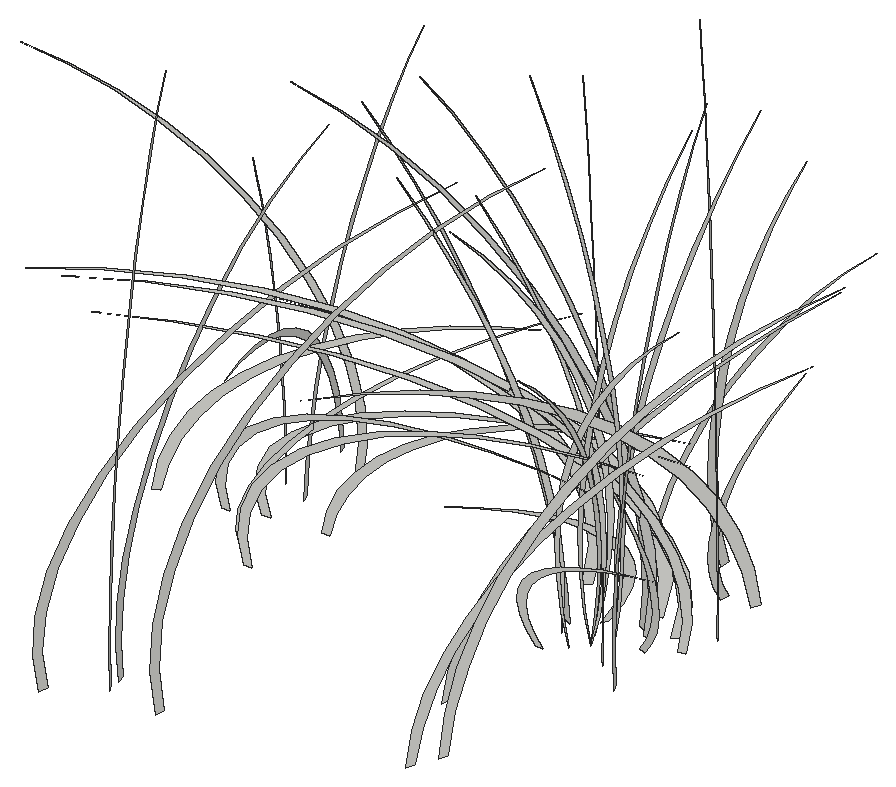
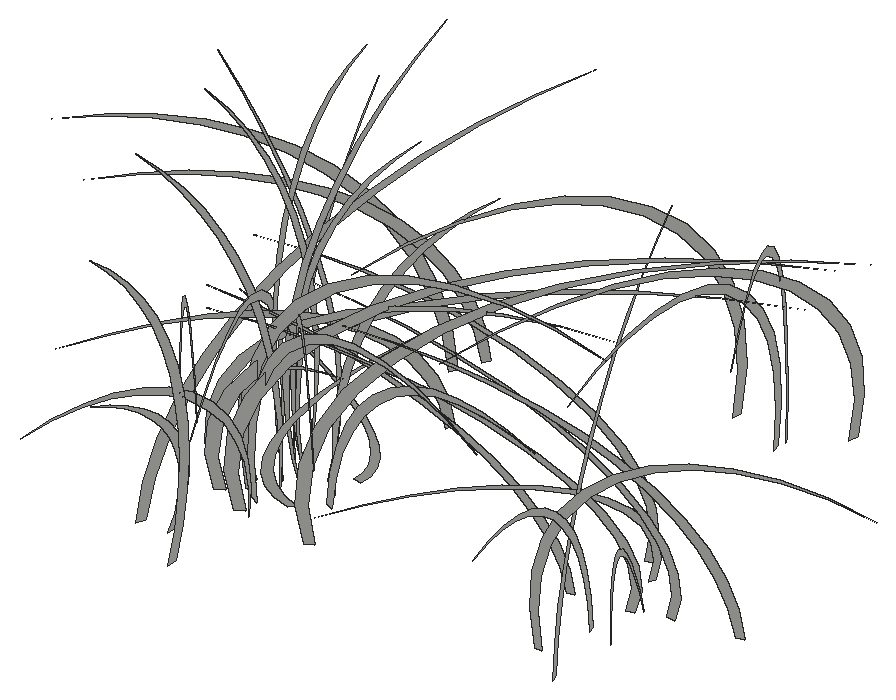
# SketchUp Ruby script. Lengths in inches.
U = 1.inch
M = Sketchup.active_model
def pt(a) = Geom::Point3d.new(a.map { |v| v * U })
def face(e, loops, mat)
  f = e.add_face(loops[0].map { |a| pt(a) })
  loops[1..].each { |l| e.add_face(l.map { |a| pt(a) }).erase! }
  f.material = f.back_material = mat if mat
  f
end
# faces: each face lists its corners as indices into pts; further lists are holes
def faces(e, pts, list, mat = nil) = list.each { |f| face(e, (f[0].is_a?(Array) ? f : [f]).map { |l| l.map { |i| pts[i] } }, mat) }
# xy, xz, yz: faces in a plane at the given z, y or x. An outline is a flat list of corners, or four numbers for a rectangle; further outlines are holes
def ring(l) = l.size == 4 ? [[l[0], l[1]], [l[2], l[1]], [l[2], l[3]], [l[0], l[3]]] : l.each_slice(2).to_a
def flat(e, list, mat, &to3) = list.each { |f| face(e, (f[0].is_a?(Array) ? f : [f]).map { |l| ring(l).map { |u, v| to3.(u, v) } }, mat) }
def xy(e, z, list, mat = nil) = flat(e, list, mat) { |x, y| [x, y, z] }
def xz(e, y, list, mat = nil) = flat(e, list, mat) { |x, z| [x, y, z] }
def yz(e, x, list, mat = nil) = flat(e, list, mat) { |y, z| [x, y, z] }
def lines(e, pts, list) = list.each { |a, b| e.add_line(pt(pts[a]), pt(pts[b])) }
# prism: a flat outline (further loops are holes) pulled along v
def prism(e, loops, v, mat = nil)
  f = face(e, loops, mat); d = Geom::Vector3d.new(v.map { |x| x * U })
  f.pushpull(f.normal.samedirection?(d) ? d.length : -d.length)
end
def box(e, o, s, mat = nil) = prism(e, [[o, [o[0] + s[0], o[1], o[2]], [o[0] + s[0], o[1] + s[1], o[2]], [o[0], o[1] + s[1], o[2]]]], [0, 0, s[2]], mat)
def at(x, y, z, deg = 0) = Geom::Transformation.translation(pt([x, y, z])) * Geom::Transformation.rotation(ORIGIN, Z_AXIS, deg.degrees)
def axes(o, x, y, z) = Geom::Transformation.new([*x, 0, *y, 0, *z, 0, *pt(o).to_a, 1])
def part(name) = M.definitions.add(name)
# library, detail: a bought-in or finely detailed component or shape, given as its bounding box
def library(name, o, s) = part(name).tap { |d| box(d.entities, o, s) }
def detail(e, o, s) = box(e.add_group.entities, o, s)
def put(e, d, t, mat = nil) = e.add_instance(d, t).tap { |i| i.material = mat if mat }
def group(e, t, mat = nil) = e.add_group.tap { |g| g.transformation = t; g.material = mat if mat }.entities
root = M.entities
g1 = group(root,at(67.39,563.36,0.02))
p = [[-0.5,0.78,0],[-0.22,0.34,0],[0,0,2.37],[-0.09,0.14,4.75],[-0.49,0.76,7.08],[-1.2,1.84,9.32],
  [-2.1875,3.37,11.39],[-3.4375,5.29,13.25],[-4.92,7.57,14.85],[-6.59,10.14,16.15],[-8.41,12.95,17.13],[-10.34,15.92,17.75],
  [-12.32,18.97,18.01],[-14.32,22.05,17.89],[-12.36,19.03,17.91],[-10.42,16.05,17.58],[-8.55,13.16,16.9],[-6.78,10.45,15.89],
  [-5.17,7.96,14.58],[-3.73,5.75,12.99],[-2.52,3.88,11.15],[-1.55,2.39,9.125],[-0.86,1.32,6.94],[-0.44,0.68,4.66],
  [-0.33,0.5,2.33]]
faces(g1,p,[[0,1,2,3,4,5,6,7,8,9,10,11,12,13,14,15,16,17,18,19,20,21,22,23,24]])
g2 = group(root,at(64.68,561.18,0.02))
p = [[0.08,0.99,0],[0.03,0.44,0],[0,0,2.01],[0.01,0.18,4.04],[0.08,0.97,6.02],[0.19,2.35,7.92],
  [0.34,4.3,9.68],[0.53,6.75,11.26],[0.76,9.66,12.62],[1.02,12.94,13.73],[1.3,16.52,14.5625],[1.6,20.31,15.09],
  [1.91,24.21,15.31],[2.21,28.13,15.2],[1.91,24.29,15.22],[1.61,20.48,14.94],[1.32,16.8,14.37],[1.05,13.33,13.51],
  [0.8,10.15,12.39],[0.58,7.34,11.04],[0.39,4.95,9.48],[0.24,3.05,7.75],[0.13,1.68,5.9],[0.07,0.87,3.96],
  [0.05,0.64,1.98]]
faces(g2,p,[[0,1,2,3,4,5,6,7,8,9,10,11,12,13,14,15,16,17,18,19,20,21,22,23,24]])
g3 = group(root,at(70.15,562.89,0.02))
p = [[0.07,0.92,0],[0.03,0.41,0],[0,0,2.37],[0.01,0.17,4.75],[0.07,0.9,7.08],[0.17,2.19,9.32],
  [0.32,4,11.39],[0.5,6.29,13.25],[0.71,9,14.85],[0.95,12.06,16.15],[1.21,15.39,17.13],[1.49,18.92,17.75],
  [1.78,22.55,18.01],[2.0625,26.21,17.89],[1.78,22.625,17.91],[1.5,19.08,17.58],[1.23,15.65,16.9],[0.98,12.42,15.89],
  [0.74,9.46,14.58],[0.54,6.84,12.99],[0.36,4.61,11.15],[0.22,2.84,9.125],[0.125,1.57,6.94],[0.0625,0.8125,4.66],
  [0.05,0.59,2.33]]
faces(g3,p,[[0,1,2,3,4,5,6,7,8,9,10,11,12,13,14,15,16,17,18,19,20,21,22,23,24]])
g4 = group(root,at(82.15,566.53,0.02))
p = [[7.01,17,14.81],[8.0625,19.56,15.2],[7.04,17.08,14.73],[6.05,14.68,14.07],[5.11,12.39,13.24],[4.22,10.24,12.25],
  [3.4,8.26,11.1],[2.66,6.45,9.81],[2,4.85,8.39],[1.43,3.47,6.86],[0.96,2.33,5.24],[0.59,1.4375,3.55],
  [0.33,0.81,1.79],[0.18,0.44,0],[0,0,0],[0.125,0.3,1.83],[0.37,0.89,3.63],[0.73,1.77,5.37],
  [1.2,2.92,7.03],[1.78,4.32,8.59],[2.46,5.97,10.02],[3.23,7.84,11.32],[4.08,9.91,12.46],[5,12.14,13.43],
  [5.98,14.51,14.21]]
faces(g4,p,[[0,1,2,3,4,5,6,7,8,9,10,11,12,13,14,15,16,17,18,19,20,21,22,23,24]])
g5 = group(root,at(67.11,564.21,0.02))
p = [[-0.27,0.88,0],[-0.12,0.39,0],[0,0,2.0625],[-0.05,0.16,4.13],[-0.26,0.87,6.16],[-0.64,2.1,8.1],
  [-1.17,3.84,9.91],[-1.84,6.03,11.52],[-2.64,8.63,12.92],[-3.54,11.5625,14.05],[-4.51,14.76,14.9],[-5.55,18.15,15.45],
  [-6.61,21.64,15.67],[-7.69,25.14,15.5625],[-6.63,21.7,15.58],[-5.59,18.3,15.29],[-4.59,15.01,14.71],[-3.64,11.91,13.83],
  [-2.77,9.07,12.68],[-2,6.56,11.3],[-1.35,4.43,9.7],[-0.83,2.73,7.9375],[-0.46,1.5,6.04],[-0.24,0.78,4.05],
  [-0.17,0.57,2.02]]
faces(g5,p,[[0,1,2,3,4,5,6,7,8,9,10,11,12,13,14,15,16,17,18,19,20,21,22,23,24]])
g6 = group(root,at(85.34,588.43,0.02))
p = [[-7.92,-19.21,16.73],[-9.11,-22.11,17.17],[-7.96,-19.3,16.64],[-6.84,-16.59,15.9],[-5.77,-14.01,14.96],[-4.77,-11.58,13.84],
  [-3.85,-9.33,12.54],[-3,-7.29,11.08],[-2.26,-5.48,9.48],[-1.62,-3.92,7.76],[-1.09,-2.63,5.92],[-0.67,-1.625,4.01],
  [-0.375,-0.91,2.02],[-0.21,-0.5,0],[0,0,0],[-0.14,-0.34,2.07],[-0.41,-1.01,4.1],[-0.82,-2,6.07],
  [-1.36,-3.3,7.94],[-2.01,-4.89,9.7],[-2.78,-6.75,11.33],[-3.65,-8.86,12.79],[-4.61,-11.19,14.08],[-5.65,-13.72,15.17],
  [-6.76,-16.4,16.0625]]
faces(g6,p,[[0,1,2,3,4,5,6,7,8,9,10,11,12,13,14,15,16,17,18,19,20,21,22,23,24]])
g7 = group(root,at(81.5,581.54,0.02))
p = [[0.19,-0.93,0],[0.09,-0.41,1.51],[0.02,-0.1,3.03],[0,0,4.56],[0.02,-0.1,6.09],[0.08,-0.41,7.61],
  [0.19,-0.92,9.12],[0.34,-1.63,10.61],[0.53,-2.55,12.07],[0.76,-3.65,13.5],[1.02,-4.95,14.89],[1.33,-6.43,16.24],
  [1.67,-8.09,17.53],[1.35,-6.53,16.21],[1.0625,-5.13,14.86],[0.81,-3.9,13.46],[0.59,-2.85,12.03],[0.41,-1.96,10.57],
  [0.26,-1.26,9.08],[0.15,-0.75,7.58],[0.08,-0.41,6.07],[0.05,-0.26,4.55],[0.0625,-0.3,3.03],[0.11,-0.52,1.51]]
faces(g7,p,[[0,1,2,3,4,5,6,7,8,9,10,11,12,13,14,15,16,17,18,19,20,21,22,23]])
g8 = group(root,at(78.48,585.41,0.02))
p = [[-0.76,-0.53,0],[-0.34,-0.24,0],[0,0,2.0625],[-0.14,-0.1,4.13],[-0.74,-0.52,6.16],[-1.8,-1.26,8.1],
  [-3.29,-2.3,9.91],[-5.18,-3.61,11.52],[-7.4,-5.16,12.92],[-9.92,-6.92,14.05],[-12.66,-8.83,14.9],[-15.56,-10.86,15.45],
  [-18.56,-12.94,15.67],[-21.56,-15.04,15.5625],[-18.61,-12.98,15.58],[-15.69,-10.95,15.29],[-12.875,-8.98,14.71],[-10.21,-7.125,13.83],
  [-7.78,-5.43,12.68],[-5.625,-3.92,11.3],[-3.8,-2.65,9.7],[-2.34,-1.63,7.9375],[-1.29,-0.9,6.04],[-0.67,-0.47,4.05],
  [-0.49,-0.34,2.02]]
faces(g8,p,[[0,1,2,3,4,5,6,7,8,9,10,11,12,13,14,15,16,17,18,19,20,21,22,23,24]])
g9 = group(root,at(78.48,585.41,0.02))
p = [[-0.76,-0.53,0],[-0.34,-0.24,0],[0,0,2.0625],[-0.14,-0.1,4.13],[-0.74,-0.52,6.16],[-1.8,-1.26,8.1],
  [-3.29,-2.3,9.91],[-5.18,-3.61,11.52],[-7.4,-5.16,12.92],[-9.92,-6.92,14.05],[-12.66,-8.83,14.9],[-15.56,-10.86,15.45],
  [-18.56,-12.94,15.67],[-21.56,-15.04,15.5625],[-18.61,-12.98,15.58],[-15.69,-10.95,15.29],[-12.875,-8.98,14.71],[-10.21,-7.125,13.83],
  [-7.78,-5.43,12.68],[-5.625,-3.92,11.3],[-3.8,-2.65,9.7],[-2.34,-1.63,7.9375],[-1.29,-0.9,6.04],[-0.67,-0.47,4.05],
  [-0.49,-0.34,2.02]]
faces(g9,p,[[0,1,2,3,4,5,6,7,8,9,10,11,12,13,14,15,16,17,18,19,20,21,22,23,24]])
g10 = group(root,at(82.8,568.11,0.02))
p = [[7.01,17,18.36],[8.0625,19.56,18.85],[7.04,17.08,18.26],[6.05,14.68,17.45],[5.11,12.39,16.42],[4.22,10.24,15.1875],
  [3.4,8.26,13.76],[2.66,6.45,12.16],[2,4.85,10.41],[1.43,3.47,8.51],[0.96,2.33,6.5],[0.59,1.4375,4.4],
  [0.33,0.81,2.22],[0.18,0.44,0],[0,0,0],[0.125,0.3,2.27],[0.37,0.89,4.5],[0.73,1.77,6.66],
  [1.2,2.92,8.72],[1.78,4.32,10.65],[2.46,5.97,12.43],[3.23,7.84,14.04],[4.08,9.91,15.45],[5,12.14,16.65],
  [5.98,14.51,17.625]]
faces(g10,p,[[0,1,2,3,4,5,6,7,8,9,10,11,12,13,14,15,16,17,18,19,20,21,22,23,24]])
g11 = group(root,at(64.3125,576.6,0.02))
p = [[0.76,0.1,0],[0.34,0.04,0],[0,0,1.44],[0.14,0.02,2.89],[0.74,0.09,4.3125],[1.8,0.23,5.67],
  [3.28,0.41,6.93],[5.15,0.65,8.0625],[7.37,0.93,9.04],[9.875,1.24,9.83],[12.61,1.59,10.43],[15.5,1.95,10.81],
  [18.47,2.33,10.96],[21.46,2.7,10.89],[18.53,2.33,10.9],[15.625,1.97,10.7],[12.82,1.61,10.29],[10.17,1.28,9.67],
  [7.75,0.98,8.875],[5.6,0.71,7.9],[3.78,0.48,6.79],[2.33,0.29,5.55],[1.28,0.16,4.22],[0.66,0.08,2.83],
  [0.49,0.0625,1.42]]
faces(g11,p,[[0,1,2,3,4,5,6,7,8,9,10,11,12,13,14,15,16,17,18,19,20,21,22,23,24]])
g12 = group(root,at(84.95,583.91,0.02))
p = [[-0.9,-0.41,0],[-0.4,-0.18,0],[0,0,1.75],[-0.16,-0.07,3.51],[-0.89,-0.4,5.24],[-2.15,-0.97,6.89],
  [-3.93,-1.77,8.42],[-6.17,-2.79,9.8],[-8.83,-3.99,10.98],[-11.83,-5.34,11.95],[-15.1,-6.82,12.67],[-18.57,-8.38,13.13],
  [-22.14,-9.99,13.32],[-25.72,-11.61,13.23],[-22.2,-10.03,13.25],[-18.72,-8.45,13],[-15.36,-6.93,12.5],[-12.1875,-5.5,11.75],
  [-9.28,-4.19,10.78],[-6.71,-3.03,9.6],[-4.53,-2.04,8.25],[-2.79,-1.26,6.75],[-1.54,-0.69,5.13],[-0.8,-0.36,3.44],
  [-0.58,-0.26,1.72]]
faces(g12,p,[[0,1,2,3,4,5,6,7,8,9,10,11,12,13,14,15,16,17,18,19,20,21,22,23,24]])
g13 = group(root,at(83.01,584.91,0.02))
p = [[-0.87,-0.48,0],[-0.39,-0.21,0],[0,0,2.01],[-0.16,-0.09,4.04],[-0.85,-0.47,6.02],[-2.07,-1.13,7.92],
  [-3.78,-2.07,9.68],[-5.94,-3.25,11.26],[-8.5,-4.65,12.62],[-11.39,-6.23,13.73],[-14.54,-7.96,14.5625],[-17.87,-9.78,15.09],
  [-21.3,-11.66,15.31],[-24.75,-13.55,15.2],[-21.37,-11.7,15.22],[-18.02,-9.86,14.94],[-14.78,-8.09,14.37],[-11.73,-6.42,13.51],
  [-8.93,-4.89,12.39],[-6.46,-3.53,11.04],[-4.36,-2.39,9.48],[-2.6875,-1.47,7.75],[-1.48,-0.8125,5.9],[-0.77,-0.42,3.96],
  [-0.5625,-0.31,1.98]]
faces(g13,p,[[0,1,2,3,4,5,6,7,8,9,10,11,12,13,14,15,16,17,18,19,20,21,22,23,24]])
g14 = group(root,at(78.45,579.32,0.02))
p = [[9.36,-1.55,6.7],[7.58,-1.26,6.27],[5.97,-0.99,5.81],[4.55,-0.76,5.31],[3.33,-0.55,4.77],[2.32,-0.38,4.21],
  [1.52,-0.25,3.63],[0.96,-0.16,3.03],[0.63,-0.1,2.43],[0.53,-0.09,1.8125],[0.67,-0.11,1.2],[1.05,-0.17,0.59],
  [1.66,-0.28,0],[1.25,-0.21,0],[0.5625,-0.09,0.59],[0.12,-0.02,1.19],[-0.06,0.01,1.81],[0.02,0,2.43],
  [0.36,-0.06,3.04],[0.96,-0.16,3.65],[1.8,-0.3,4.23],[2.89,-0.48,4.8],[4.2,-0.7,5.33],[5.73,-0.95,5.83],
  [7.46,-1.24,6.29]]
faces(g14,p,[[0,1,2,3,4,5,6,7,8,9,10,11,12,13,14,15,16,17,18,19,20,21,22,23,24]])
g15 = group(root,at(81.6,582.35,0.02))
p = [[-0.41,-0.86,0],[-0.18,-0.38,1.97],[-0.05,-0.1,3.96],[0,0,5.95],[-0.04,-0.09,7.95],[-0.18,-0.38,9.9375],
  [-0.4,-0.85,11.91],[-0.72,-1.51,13.85],[-1.12,-2.35,15.76],[-1.61,-3.37,17.63],[-2.18,-4.5625,19.44],[-2.83,-5.93,21.2],
  [-3.56,-7.46,22.89],[-2.87,-6.02,21.17],[-2.26,-4.73,19.4],[-1.72,-3.6,17.58],[-1.25,-2.62,15.71],[-0.86,-1.8125,13.8],
  [-0.56,-1.16,11.86],[-0.33,-0.6875,9.9],[-0.18,-0.38,7.93],[-0.11,-0.24,5.94],[-0.13,-0.27,3.95],[-0.23,-0.48,1.97]]
faces(g15,p,[[0,1,2,3,4,5,6,7,8,9,10,11,12,13,14,15,16,17,18,19,20,21,22,23]])
g16 = group(root,at(61.38,588,0.02))
p = [[6.57,-15.79,13.77],[7.5625,-18.17,14.14],[6.6,-15.86,13.7],[5.68,-13.63,13.09],[4.79,-11.51,12.32],[3.96,-9.51,11.39],
  [3.19,-7.67,10.32],[2.49,-5.99,9.12],[1.875,-4.5,7.8],[1.34,-3.22,6.38],[0.9,-2.16,4.875],[0.56,-1.34,3.3],
  [0.3125,-0.75,1.67],[0.17,-0.41,0],[0,0,0],[0.12,-0.28,1.71],[0.34,-0.83,3.38],[0.68,-1.64,4.99],
  [1.13,-2.71,6.54],[1.67,-4.02,7.99],[2.31,-5.55,9.32],[3.03,-7.28,10.53],[3.83,-9.2,11.59],[4.69,-11.27,12.49],
  [5.61,-13.48,13.22]]
faces(g16,p,[[0,1,2,3,4,5,6,7,8,9,10,11,12,13,14,15,16,17,18,19,20,21,22,23,24]])
g17 = group(root,at(80.06,580.01,0.02))
p = [[0.9375,-0.14,0],[0.42,-0.06,1.67],[0.11,-0.02,3.36],[0,0,5.0625],[0.1,-0.01,6.76],[0.41,-0.06,8.45],
  [0.93,-0.13,10.12],[1.65,-0.24,11.77],[2.57,-0.37,13.4],[3.69,-0.53,14.98],[5,-0.72,16.53],[6.5,-0.9375,18.02],
  [8.18,-1.18,19.46],[6.6,-0.95,18],[5.1875,-0.75,16.49],[3.94,-0.57,14.9375],[2.875,-0.42,13.35],[1.99,-0.29,11.73],
  [1.28,-0.18,10.08],[0.75,-0.11,8.42],[0.42,-0.06,6.74],[0.26,-0.04,5.05],[0.3,-0.04,3.36],[0.53,-0.08,1.68]]
faces(g17,p,[[0,1,2,3,4,5,6,7,8,9,10,11,12,13,14,15,16,17,18,19,20,21,22,23]])
g18 = group(root,at(60.17,580.18,0.02))
p = [[0.82,-0.05,0],[0.36,-0.02,0],[0,0,1.23],[0.15,-0.01,2.46],[0.8,-0.05,3.67],[1.94,-0.12,4.82],
  [3.54,-0.21,5.89],[5.56,-0.33,6.85],[7.96,-0.48,7.68],[10.66,-0.64,8.36],[13.62,-0.8125,8.86],[16.74,-1,9.18],
  [19.95,-1.19,9.32],[23.18,-1.39,9.25],[20.01,-1.2,9.27],[16.875,-1.01,9.09],[13.84,-0.83,8.74],[10.98,-0.66,8.22],
  [8.37,-0.5,7.54],[6.05,-0.36,6.72],[4.08,-0.24,5.77],[2.52,-0.15,4.72],[1.39,-0.08,3.59],[0.72,-0.04,2.41],
  [0.53,-0.03,1.2]]
faces(g18,p,[[0,1,2,3,4,5,6,7,8,9,10,11,12,13,14,15,16,17,18,19,20,21,22,23,24]])
g19 = group(root,at(81.42,584.09,0.02))
p = [[-4.26,-8.48,7.88],[-3.45,-6.87,7.38],[-2.72,-5.41,6.83],[-2.07,-4.12,6.24],[-1.52,-3.01,5.62],[-1.06,-2.1,4.96],
  [-0.69,-1.38,4.27],[-0.4375,-0.87,3.57],[-0.29,-0.57,2.86],[-0.24,-0.48,2.13],[-0.31,-0.61,1.41],[-0.48,-0.95,0.7],
  [-0.76,-1.5,0],[-0.57,-1.14,0],[-0.26,-0.51,0.69],[-0.05,-0.11,1.4],[0.03,0.05,2.13],[-0.01,-0.02,2.85],
  [-0.16,-0.33,3.58],[-0.44,-0.87,4.29],[-0.82,-1.63,4.98],[-1.32,-2.62,5.64],[-1.91,-3.81,6.27],[-2.61,-5.19,6.86],
  [-3.4,-6.75,7.4]]
faces(g19,p,[[0,1,2,3,4,5,6,7,8,9,10,11,12,13,14,15,16,17,18,19,20,21,22,23,24]])
g20 = group(root,at(82.64,580.52,0.02))
p = [[-0.94,0.09,0],[-0.42,0.04,1.77],[-0.11,0.01,3.57],[0,0,5.36],[-0.1,0.01,7.16],[-0.42,0.04,8.95],
  [-0.9375,0.09,10.73],[-1.66,0.16,12.48],[-2.59,0.25,14.2],[-3.71,0.36,15.88],[-5.03,0.49,17.52],[-6.54,0.64,19.1],
  [-8.23,0.81,20.625],[-6.64,0.65,19.08],[-5.22,0.51,17.48],[-3.97,0.39,15.83],[-2.89,0.28,14.15],[-2,0.2,12.43],
  [-1.28,0.125,10.6875],[-0.76,0.07,8.92],[-0.42,0.04,7.14],[-0.27,0.03,5.35],[-0.3,0.03,3.5625],[-0.53,0.05,1.78]]
faces(g20,p,[[0,1,2,3,4,5,6,7,8,9,10,11,12,13,14,15,16,17,18,19,20,21,22,23]])
g21 = group(root,at(85.82,582.81,0.02))
p = [[-0.75,-0.12,0],[-0.33,-0.05,0],[0,0,1.68],[-0.13,-0.02,3.37],[-0.73,-0.12,5.03],[-1.78,-0.29,6.61],
  [-3.25,-0.53,8.08],[-5.11,-0.84,9.4],[-7.3,-1.2,10.54],[-9.79,-1.6,11.47],[-12.49,-2.05,12.16],[-15.36,-2.51,12.61],
  [-18.31,-3,12.79],[-21.27,-3.48,12.7],[-18.36,-3.01,12.72],[-15.49,-2.54,12.48],[-12.7,-2.08,12],[-10.08,-1.65,11.29],
  [-7.68,-1.26,10.35],[-5.55,-0.91,9.22],[-3.75,-0.61,7.92],[-2.31,-0.38,6.48],[-1.27,-0.21,4.93],[-0.66,-0.11,3.31],
  [-0.48,-0.08,1.65]]
faces(g21,p,[[0,1,2,3,4,5,6,7,8,9,10,11,12,13,14,15,16,17,18,19,20,21,22,23,24]])
g22 = group(root,at(79.99,580.78,0.02))
p = [[-10.57,1.04,19.61],[-8.88,0.87,18.16],[-7.34,0.72,16.67],[-5.93,0.58,15.125],[-4.67,0.46,13.55],[-3.55,0.35,11.93],
  [-2.59,0.25,10.28],[-1.79,0.18,8.61],[-1.14,0.11,6.91],[-0.65,0.0625,5.2],[-0.32,0.03,3.47],[-0.15,0.01,1.74],
  [-0.14,0.01,0],[0,0,1.74],[-0.05,0.01,3.49],[-0.29,0.03,5.23],[-0.72,0.07,6.96],[-1.33,0.13,8.67],
  [-2.13,0.21,10.36],[-3.11,0.31,12.01],[-4.27,0.42,13.63],[-5.6,0.55,15.21],[-7.09,0.7,16.73],[-8.75,0.86,18.2]]
faces(g22,p,[[0,1,2,3,4,5,6,7,8,9,10,11,12,13,14,15,16,17,18,19,20,21,22,23]])
g23 = group(root,at(79.99,580.78,0.02))
p = [[-10.57,1.04,19.61],[-8.88,0.87,18.16],[-7.34,0.72,16.67],[-5.93,0.58,15.125],[-4.67,0.46,13.55],[-3.55,0.35,11.93],
  [-2.59,0.25,10.28],[-1.79,0.18,8.61],[-1.14,0.11,6.91],[-0.65,0.0625,5.2],[-0.32,0.03,3.47],[-0.15,0.01,1.74],
  [-0.14,0.01,0],[0,0,1.74],[-0.05,0.01,3.49],[-0.29,0.03,5.23],[-0.72,0.07,6.96],[-1.33,0.13,8.67],
  [-2.13,0.21,10.36],[-3.11,0.31,12.01],[-4.27,0.42,13.63],[-5.6,0.55,15.21],[-7.09,0.7,16.73],[-8.75,0.86,18.2]]
faces(g23,p,[[0,1,2,3,4,5,6,7,8,9,10,11,12,13,14,15,16,17,18,19,20,21,22,23]])
g24 = group(root,at(62.02,580.72,0.02))
p = [[0.8125,0.1,0],[0.36,0.05,0],[0,0,1.23],[0.15,0.02,2.46],[0.79,0.1,3.67],[1.93,0.24,4.82],
  [3.52,0.44,5.89],[5.53,0.7,6.85],[7.91,1,7.68],[10.6,1.34,8.36],[13.53,1.7,8.86],[16.64,2.1,9.18],
  [19.83,2.5,9.32],[23.04,2.9,9.25],[19.89,2.51,9.27],[16.77,2.11,9.09],[13.76,1.73,8.74],[10.92,1.375,8.22],
  [8.31,1.05,7.54],[6.01,0.76,6.72],[4.06,0.51,5.77],[2.5,0.32,4.72],[1.38,0.17,3.59],[0.71,0.09,2.41],
  [0.52,0.07,1.2]]
faces(g24,p,[[0,1,2,3,4,5,6,7,8,9,10,11,12,13,14,15,16,17,18,19,20,21,22,23,24]])
g25 = group(root,at(83.42,580.875,0.02))
p = [[-0.89,0.32,0],[-0.4,0.14,2.26],[-0.1,0.04,4.55],[0,0,6.84],[-0.1,0.04,9.14],[-0.39,0.14,11.42],
  [-0.88,0.32,13.6875],[-1.57,0.57,15.92],[-2.45,0.89,18.12],[-3.51,1.27,20.26],[-4.75,1.72,22.35],[-6.18,2.24,24.37],
  [-7.77,2.8125,26.3125],[-6.27,2.27,24.34],[-4.93,1.78,22.3],[-3.75,1.36,20.2],[-2.73,0.99,18.05],[-1.89,0.68,15.86],
  [-1.21,0.4375,13.64],[-0.72,0.26,11.38],[-0.39,0.14,9.11],[-0.25,0.09,6.83],[-0.29,0.1,4.54],[-0.5,0.18,2.27]]
faces(g25,p,[[0,1,2,3,4,5,6,7,8,9,10,11,12,13,14,15,16,17,18,19,20,21,22,23]])
g26 = group(root,at(65.54,581.16,0.02))
p = [[16.97,2.14,10.18],[19.53,2.46,10.45],[17.05,2.15,10.13],[14.65,1.85,9.68],[12.37,1.56,9.11],[10.22,1.29,8.42],
  [8.24,1.04,7.63],[6.4375,0.8125,6.75],[4.84,0.61,5.77],[3.46,0.4375,4.72],[2.33,0.29,3.61],[1.4375,0.18,2.4375],
  [0.81,0.1,1.23],[0.44,0.06,0],[0,0,0],[0.3,0.04,1.26],[0.89,0.11,2.5],[1.76,0.22,3.69],
  [2.91,0.37,4.83],[4.32,0.54,5.91],[5.96,0.75,6.89],[7.83,0.99,7.78],[9.89,1.25,8.57],[12.11,1.53,9.24],
  [14.48,1.82,9.78]]
faces(g26,p,[[0,1,2,3,4,5,6,7,8,9,10,11,12,13,14,15,16,17,18,19,20,21,22,23,24]])
g27 = group(root,at(56.93,579.57,0.02))
p = [[16.35,5,11.98],[18.82,5.75,12.3],[16.43,5.02,11.91],[14.12,4.32,11.39],[11.92,3.65,10.71],[9.85,3.01,9.91],
  [7.94,2.43,8.98],[6.21,1.9,7.9375],[4.67,1.43,6.79],[3.34,1.02,5.55],[2.24,0.69,4.24],[1.38,0.42,2.87],
  [0.78,0.24,1.45],[0.43,0.13,0],[0,0,0],[0.29,0.09,1.48],[0.86,0.26,2.9375],[1.7,0.52,4.35],
  [2.81,0.86,5.6875],[4.16,1.27,6.95],[5.75,1.76,8.11],[7.54,2.31,9.16],[9.53,2.91,10.08],[11.68,3.57,10.87],
  [13.96,4.27,11.5]]
faces(g27,p,[[0,1,2,3,4,5,6,7,8,9,10,11,12,13,14,15,16,17,18,19,20,21,22,23,24]])
g28 = group(root,at(85.13,581.22,0.02))
p = [[-8.86,3.42,9.0625],[-7.17,2.77,8.49],[-5.65,2.18,7.85],[-4.3,1.66,7.18],[-3.15,1.21,6.45],[-2.19,0.85,5.7],
  [-1.44,0.56,4.91],[-0.91,0.35,4.1],[-0.6,0.23,3.28],[-0.5,0.19,2.45],[-0.64,0.25,1.625],[-0.99,0.38,0.8],
  [-1.57,0.61,0],[-1.1875,0.46,0],[-0.53,0.2,0.8],[-0.11,0.04,1.61],[0.06,-0.02,2.45],[-0.02,0.01,3.28],
  [-0.34,0.13,4.11],[-0.9,0.35,4.93],[-1.7,0.66,5.72],[-2.73,1.05,6.49],[-3.98,1.53,7.21],[-5.42,2.09,7.88],
  [-7.05,2.72,8.5]]
faces(g28,p,[[0,1,2,3,4,5,6,7,8,9,10,11,12,13,14,15,16,17,18,19,20,21,22,23,24]])
g29 = group(root,at(81.69,579.66,0.02))
yz(g29,0,[[0.95,0,0.42,2.04,0.11,4.1,0,6.17,0.1,8.23,0.42,10.29,0.94,12.33,1.67,14.34,2.6,16.32,3.73,18.26,5.06,20.14,6.57,21.96,8.26,23.71,6.67,21.93,5.24,20.09,3.99,18.2,2.91,16.26,2.01,14.29,1.29,12.29,0.76,10.26,0.42,8.21,0.27,6.15,0.3,4.09,0.53,2.04]])
g30 = group(root,at(79.7,572.22,0.02))
p = [[3.87,20.41,12.375],[4.45,23.49,12.7],[3.88,20.51,12.31],[3.34,17.63,11.76],[2.82,14.88,11.07],[2.33,12.3,10.23],
  [1.88,9.91,9.27],[1.47,7.75,8.2],[1.1,5.82,7.01],[0.79,4.17,5.74],[0.53,2.8,4.38],[0.33,1.73,2.96],
  [0.18,0.97,1.5],[0.1,0.53,0],[0,0,0],[0.07,0.36,1.53],[0.2,1.07,3.03],[0.4,2.12,4.49],
  [0.66,3.5,5.875],[0.98,5.19,7.18],[1.36,7.17,8.375],[1.78,9.42,9.46],[2.25,11.89,10.41],[2.76,14.58,11.22],
  [3.3,17.43,11.88]]
faces(g30,p,[[0,1,2,3,4,5,6,7,8,9,10,11,12,13,14,15,16,17,18,19,20,21,22,23,24]])
g31 = group(root,at(83.87,582.67,0.02))
p = [[-0.9,0.19,0],[-0.4,0.09,0],[0,0,2.37],[-0.16,0.03,4.75],[-0.89,0.1875,7.08],[-2.15,0.46,9.32],
  [-3.93,0.83,11.39],[-6.17,1.3125,13.25],[-8.83,1.875,14.85],[-11.83,2.51,16.15],[-15.1,3.21,17.13],[-18.5625,3.95,17.75],
  [-22.13,4.7,18.01],[-25.71,5.47,17.89],[-22.2,4.72,17.91],[-18.72,3.98,17.58],[-15.35,3.26,16.9],[-12.18,2.59,15.89],
  [-9.28,1.97,14.58],[-6.71,1.43,12.99],[-4.53,0.96,11.15],[-2.79,0.59,9.125],[-1.54,0.33,6.94],[-0.8,0.17,4.66],
  [-0.58,0.125,2.33]]
faces(g31,p,[[0,1,2,3,4,5,6,7,8,9,10,11,12,13,14,15,16,17,18,19,20,21,22,23,24]])
g32 = group(root,at(63.45,577.5,0.02))
p = [[0.25,0.57,0],[0.11,0.25,0],[0,0,1.02],[0.05,0.1,2.05],[0.25,0.56,3.0625],[0.6,1.36,4.03],
  [1.1,2.48,4.92],[1.73,3.89,5.72],[2.48,5.5625,6.42],[3.32,7.45,6.98],[4.24,9.52,7.4],[5.21,11.7,7.67],
  [6.22,13.95,7.78],[7.22,16.2,7.73],[6.23,13.99,7.74],[5.26,11.8,7.6],[4.3125,9.68,7.3],[3.42,7.68,6.87],
  [2.61,5.85,6.3],[1.88,4.23,5.61],[1.27,2.85,4.82],[0.78,1.76,3.94],[0.43,0.97,3],[0.22,0.5,2.01],
  [0.16,0.37,1.01]]
faces(g32,p,[[0,1,2,3,4,5,6,7,8,9,10,11,12,13,14,15,16,17,18,19,20,21,22,23,24]])
g33 = group(root,at(64.27,586.0625,0.02))
p = [[-0.76,0.06,0],[-0.34,0.03,0],[0,0,1.95],[-0.14,0.01,3.91],[-0.74,0.06,5.83],[-1.8,0.14,7.67],
  [-3.29,0.26,9.37],[-5.18,0.41,10.9],[-7.4,0.58,12.22],[-9.92,0.78,13.3],[-12.67,1,14.1],[-15.57,1.23,14.61],
  [-18.5625,1.46,14.82],[-21.57,1.7,14.72],[-18.62,1.47,14.74],[-15.7,1.24,14.47],[-12.88,1.01,13.91],[-10.22,0.8,13.08],
  [-7.78,0.61,12],[-5.625,0.44,10.6875],[-3.8,0.3,9.18],[-2.34,0.18,7.51],[-1.29,0.1,5.71],[-0.67,0.05,3.83],
  [-0.49,0.04,1.91]]
faces(g33,p,[[0,1,2,3,4,5,6,7,8,9,10,11,12,13,14,15,16,17,18,19,20,21,22,23,24]])
g34 = group(root,at(79.65,581.6,0.02))
p = [[-18.35,9.75,14.56],[-21.11,11.23,14.94],[-18.43,9.8,14.48],[-15.84,8.42,13.83],[-13.375,7.11,13.02],[-11.05,5.88,12.04],
  [-8.91,4.74,10.91],[-6.96,3.7,9.64],[-5.23,2.78,8.25],[-3.75,1.99,6.75],[-2.51,1.34,5.15],[-1.55,0.83,3.49],
  [-0.87,0.46,1.76],[-0.48,0.25,0],[0,0,0],[-0.32,0.17,1.8],[-0.96,0.51,3.57],[-1.91,1.01,5.28],
  [-3.15,1.67,6.91],[-4.67,2.48,8.44],[-6.45,3.43,9.85],[-8.46,4.5,11.13],[-10.6875,5.68,12.25],[-13.1,6.97,13.2],
  [-15.66,8.33,13.97]]
faces(g34,p,[[0,1,2,3,4,5,6,7,8,9,10,11,12,13,14,15,16,17,18,19,20,21,22,23,24]])
g35 = group(root,at(81.69,582.33,0.02))
yz(g35,0,[[0.14,0,0,2.01,0.05,4.01,0.29,6.01,0.72,8,1.34,9.97,2.14,11.91,3.125,13.81,4.29,15.67,5.625,17.48,7.13,19.23,8.8,20.92,10.62,22.54,8.93,20.88,7.37,19.16,5.96,17.39,4.6875,15.57,3.57,13.71,2.6,11.82,1.79,9.89,1.14,7.94,0.65,5.97,0.32,3.99,0.15,2]])
g36 = group(root,at(61.49,583.65,0.02))
p = [[-9.78,9.78,9.36],[-8.46,8.46,9.3],[-7.17,7.17,9.07],[-5.92,5.92,8.6875],[-4.75,4.75,8.14],[-3.66,3.66,7.46],
  [-2.69,2.69,6.64],[-1.85,1.85,5.71],[-1.16,1.16,4.68],[-0.63,0.63,3.57],[-0.27,0.27,2.41],[-0.09,0.09,1.21],
  [-0.09,0.09,0],[0,0,1.23],[-0.11,0.11,2.46],[-0.43,0.43,3.67],[-0.93,0.93,4.8125],[-1.62,1.62,5.875],
  [-2.47,2.47,6.83],[-3.47,3.47,7.66],[-4.59,4.59,8.34],[-5.81,5.81,8.87],[-7.1,7.1,9.21],[-8.43,8.43,9.38]]
faces(g36,p,[[0,1,2,3,4,5,6,7,8,9,10,11,12,13,14,15,16,17,18,19,20,21,22,23]])
g37 = group(root,at(83.07,583.0625,0.02))
p = [[-0.82,0.43,0],[-0.36,0.19,0],[0,0,2.0625],[-0.15,0.08,4.13],[-0.8,0.43,6.16],[-1.94,1.03,8.1],
  [-3.55,1.89,9.91],[-5.57,2.96,11.52],[-7.97,4.24,12.92],[-10.68,5.68,14.05],[-13.63,7.25,14.9],[-16.76,8.91,15.45],
  [-19.98,10.62,15.67],[-23.21,12.34,15.5625],[-20.04,10.65,15.58],[-16.9,8.98,15.29],[-13.86,7.37,14.71],[-11,5.85,13.83],
  [-8.375,4.45,12.68],[-6.05,3.22,11.3],[-4.09,2.17,9.7],[-2.52,1.34,7.9375],[-1.39,0.74,6.04],[-0.72,0.38,4.05],
  [-0.53,0.28,2.02]]
faces(g37,p,[[0,1,2,3,4,5,6,7,8,9,10,11,12,13,14,15,16,17,18,19,20,21,22,23,24]])
g38 = group(root,at(85.29,577.6875,0.02))
p = [[-0.49,0.86,0],[-0.22,0.38,0],[0,0,2.01],[-0.09,0.15,4.04],[-0.48,0.84,6.02],[-1.18,2.05,7.92],
  [-2.15,3.74,9.68],[-3.375,5.87,11.26],[-4.83,8.4,12.62],[-6.47,11.25,13.73],[-8.26,14.37,14.5625],[-10.16,17.66,15.09],
  [-12.11,21.05,15.31],[-14.07,24.46,15.2],[-12.14,21.12,15.22],[-10.24,17.81,14.94],[-8.4,14.61,14.37],[-6.66,11.59,13.51],
  [-5.08,8.83,12.39],[-3.67,6.38,11.04],[-2.48,4.31,9.48],[-1.53,2.66,7.75],[-0.84,1.46,5.9],[-0.4375,0.76,3.96],
  [-0.32,0.56,1.98]]
faces(g38,p,[[0,1,2,3,4,5,6,7,8,9,10,11,12,13,14,15,16,17,18,19,20,21,22,23,24]])
g39 = group(root,at(83.5,579.21,0.02))
p = [[-0.64,0.76,0],[-0.29,0.34,0],[0,0,2.01],[-0.12,0.14,4.04],[-0.63,0.74,6.02],[-1.53,1.8,7.92],
  [-2.8,3.28,9.68],[-4.4,5.15,11.26],[-6.29,7.37,12.62],[-8.43,9.87,13.73],[-10.76,12.6,14.5625],[-13.23,15.49,15.09],
  [-15.77,18.47,15.31],[-18.33,21.46,15.2],[-15.82,18.52,15.22],[-13.34,15.62,14.94],[-10.94,12.8125,14.37],[-8.68,10.17,13.51],
  [-6.61,7.74,12.39],[-4.78,5.6,11.04],[-3.23,3.78,9.48],[-1.99,2.33,7.75],[-1.1,1.28,5.9],[-0.57,0.66,3.96],
  [-0.42,0.49,1.98]]
faces(g39,p,[[0,1,2,3,4,5,6,7,8,9,10,11,12,13,14,15,16,17,18,19,20,21,22,23,24]])
g40 = group(root,at(83.625,586.7,0.02))
yz(g40,0,[[0.92,0,0.43,0.81,0.12,1.65,0,2.49,0.08,3.34,0.35,4.17,0.81,4.99,1.46,5.79,2.29,6.54,3.29,7.26,4.44,7.92,5.75,8.52,7.18,9.0625,5.87,8.49,4.68,7.85,3.63,7.18,2.73,6.45,1.99,5.7,1.4,4.91,0.99,4.1,0.74,3.28,0.67,2.45,0.78,1.625,1.05,0.8,1.5,0]])
g41 = group(root,at(63.02,583.02,0.02))
p = [[-6.57,15.79,13.77],[-7.5625,18.17,14.14],[-6.6,15.86,13.7],[-5.68,13.63,13.09],[-4.79,11.51,12.32],[-3.96,9.51,11.39],
  [-3.19,7.67,10.32],[-2.49,5.99,9.12],[-1.875,4.5,7.8],[-1.34,3.22,6.38],[-0.9,2.16,4.875],[-0.56,1.34,3.3],
  [-0.3125,0.75,1.67],[-0.17,0.41,0],[0,0,0],[-0.12,0.28,1.71],[-0.34,0.83,3.38],[-0.68,1.64,4.99],
  [-1.13,2.71,6.54],[-1.67,4.02,7.99],[-2.31,5.55,9.32],[-3.03,7.28,10.53],[-3.83,9.2,11.59],[-4.69,11.27,12.49],
  [-5.61,13.48,13.22]]
faces(g41,p,[[0,1,2,3,4,5,6,7,8,9,10,11,12,13,14,15,16,17,18,19,20,21,22,23,24]])
g42 = group(root,at(81.69,589.12,0.02))
yz(g42,0,[[0.92,0,0.43,1.66,0.12,3.35,0,5.07,0.08,6.79,0.35,8.49,0.81,10.15,1.46,11.76,2.29,13.3,3.29,14.75,4.44,16.1,5.75,17.33,7.18,18.42,5.87,17.25,4.68,15.97,3.63,14.59,2.73,13.12,1.99,11.58,1.4,9.98,0.99,8.34,0.74,6.67,0.67,4.99,0.78,3.3,1.05,1.63,1.5,0]])
g43 = group(root,at(81.69,584.6,0.02))
yz(g43,0,[[0.15,0,0,1.5,0.2,3,0.74,4.46,1.6,5.85,2.78,7.14,4.25,8.3,5.96,9.31,7.89,10.14,9.98,10.77,12.2,11.19,14.49,11.4,16.8,11.375,14.54,11.3,12.32,11.03,10.18,10.55,8.15,9.89,6.29,9.0625,4.625,8.07,3.18,6.9375,1.99,5.69,1.08,4.34,0.46,2.93,0.15,1.47]])
g44 = group(root,at(86.15,584.28,0.02))
p = [[-0.6,0.7,0],[-0.27,0.3125,0],[0,0,2.37],[-0.11,0.125,4.75],[-0.59,0.6875,7.08],[-1.43,1.67,9.32],
  [-2.61,3.05,11.39],[-4.1,4.8,13.25],[-5.86,6.86,14.85],[-7.85,9.2,16.15],[-10.03,11.74,17.13],[-12.32,14.43,17.75],
  [-14.69,17.2,18.01],[-17.07,19.99,17.89],[-14.74,17.26,17.91],[-12.43,14.55,17.58],[-10.19,11.9375,16.9],[-8.09,9.47,15.89],
  [-6.16,7.21,14.58],[-4.45,5.21,12.99],[-3.01,3.52,11.15],[-1.85,2.17,9.125],[-1.02,1.2,6.94],[-0.53,0.62,4.66],
  [-0.39,0.45,2.33]]
faces(g44,p,[[0,1,2,3,4,5,6,7,8,9,10,11,12,13,14,15,16,17,18,19,20,21,22,23,24]])
